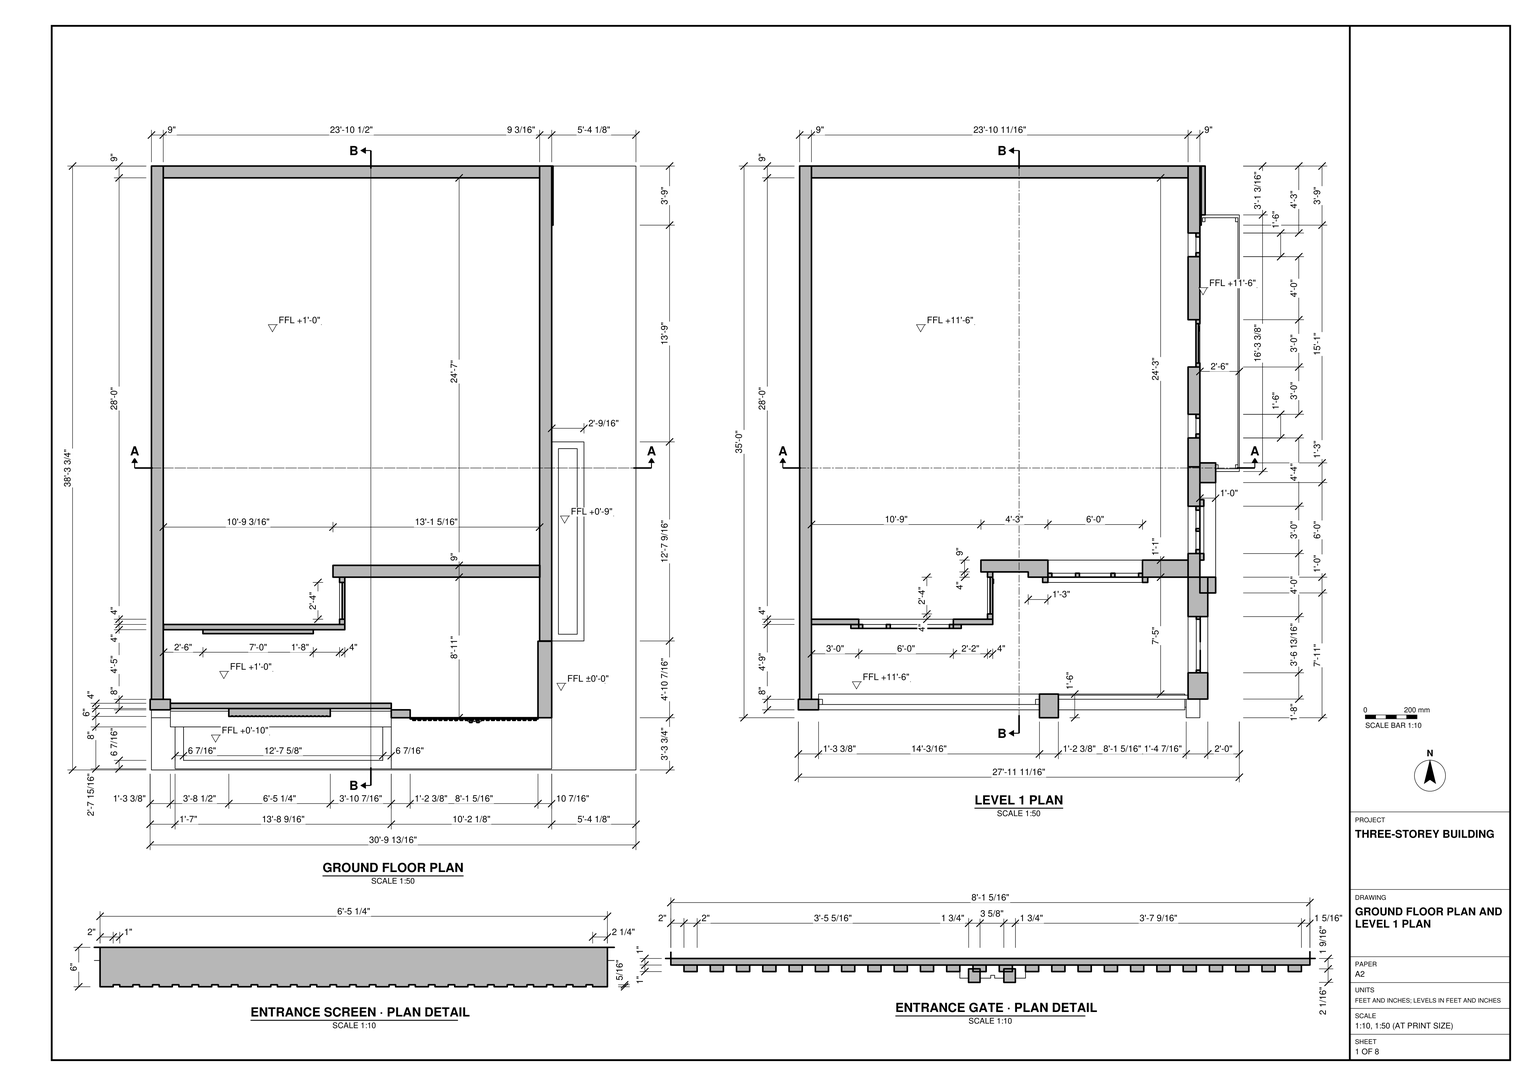
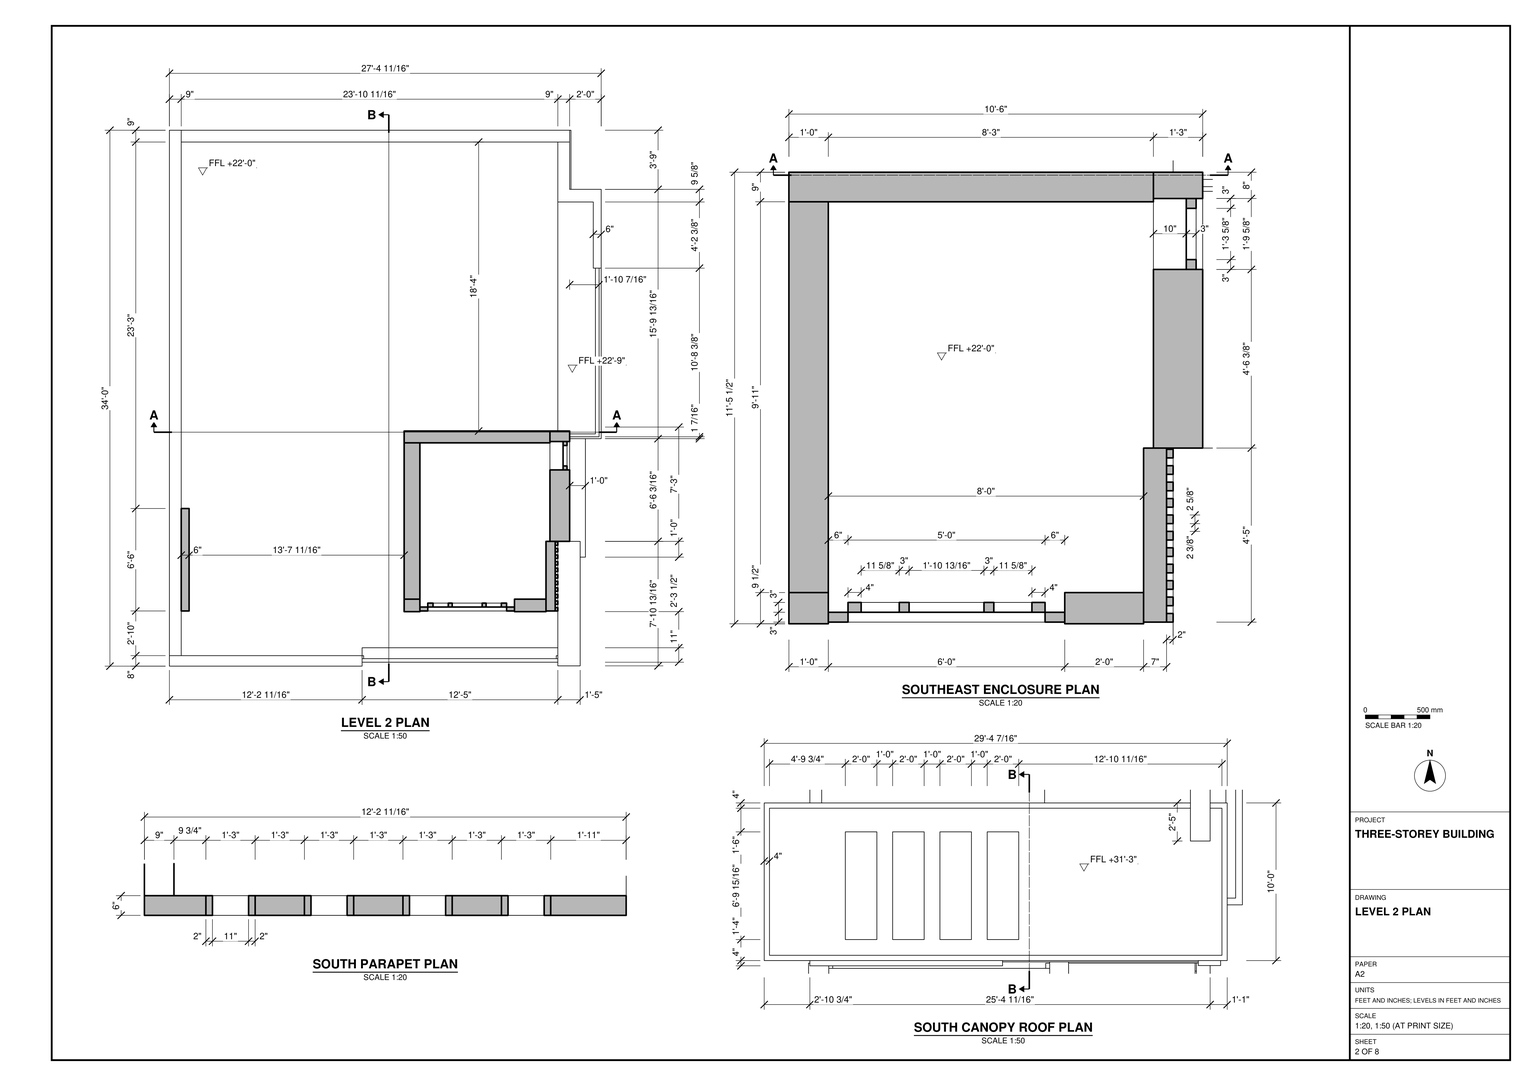
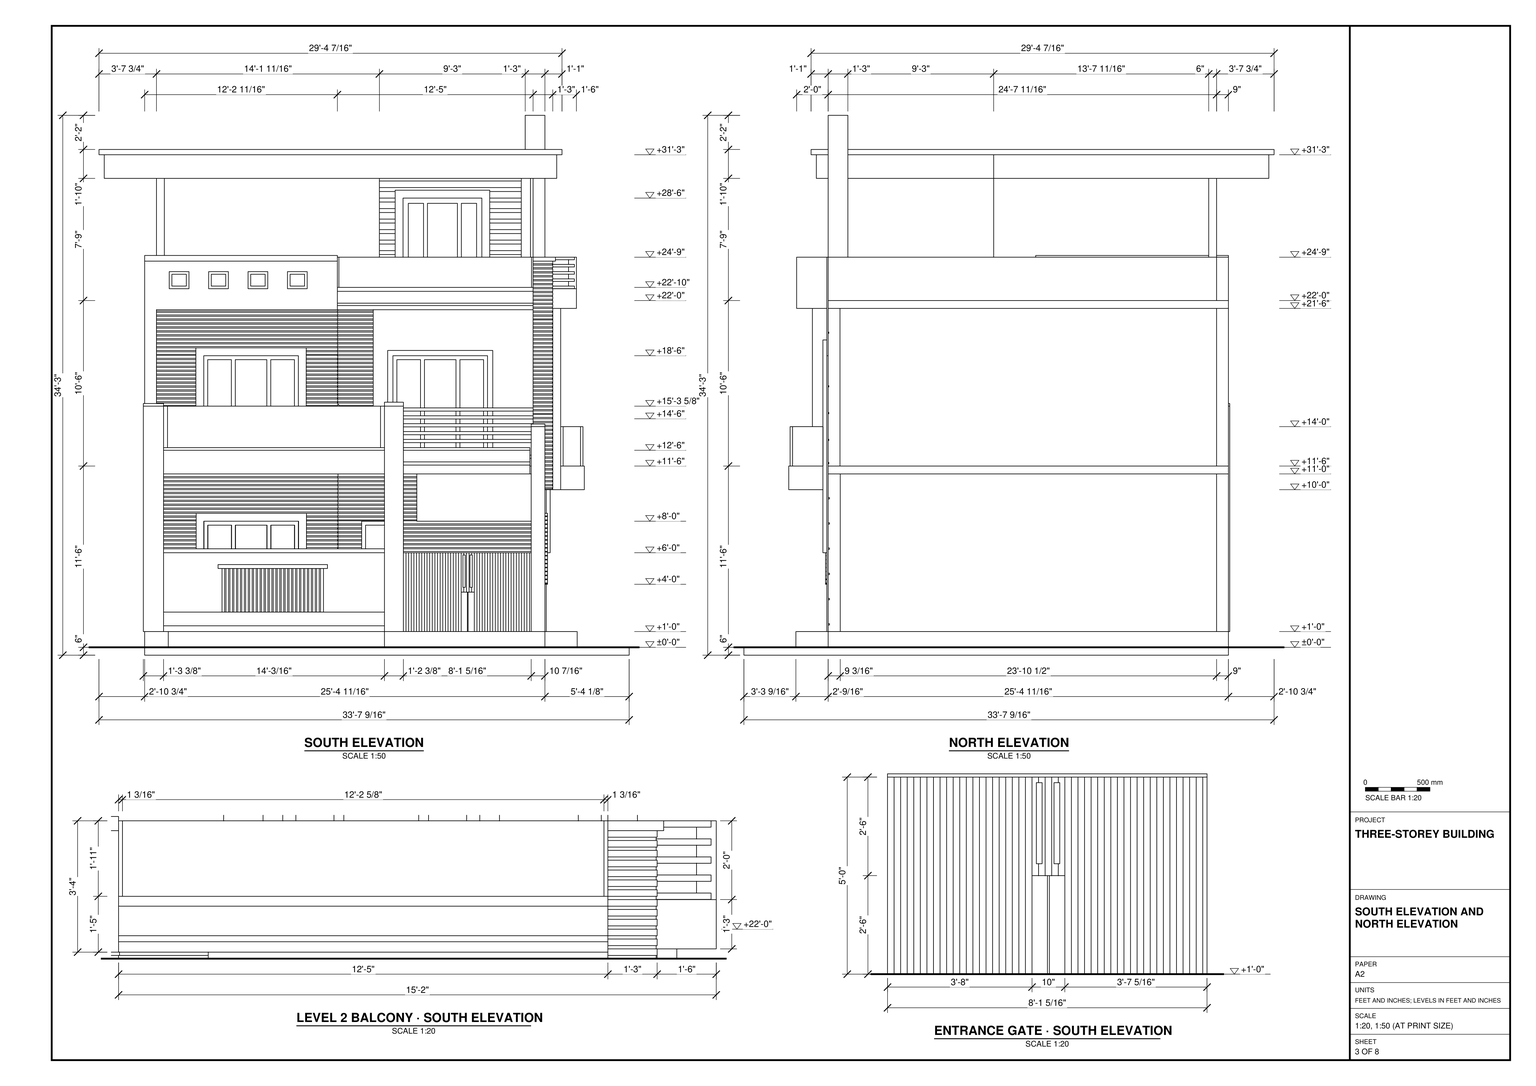
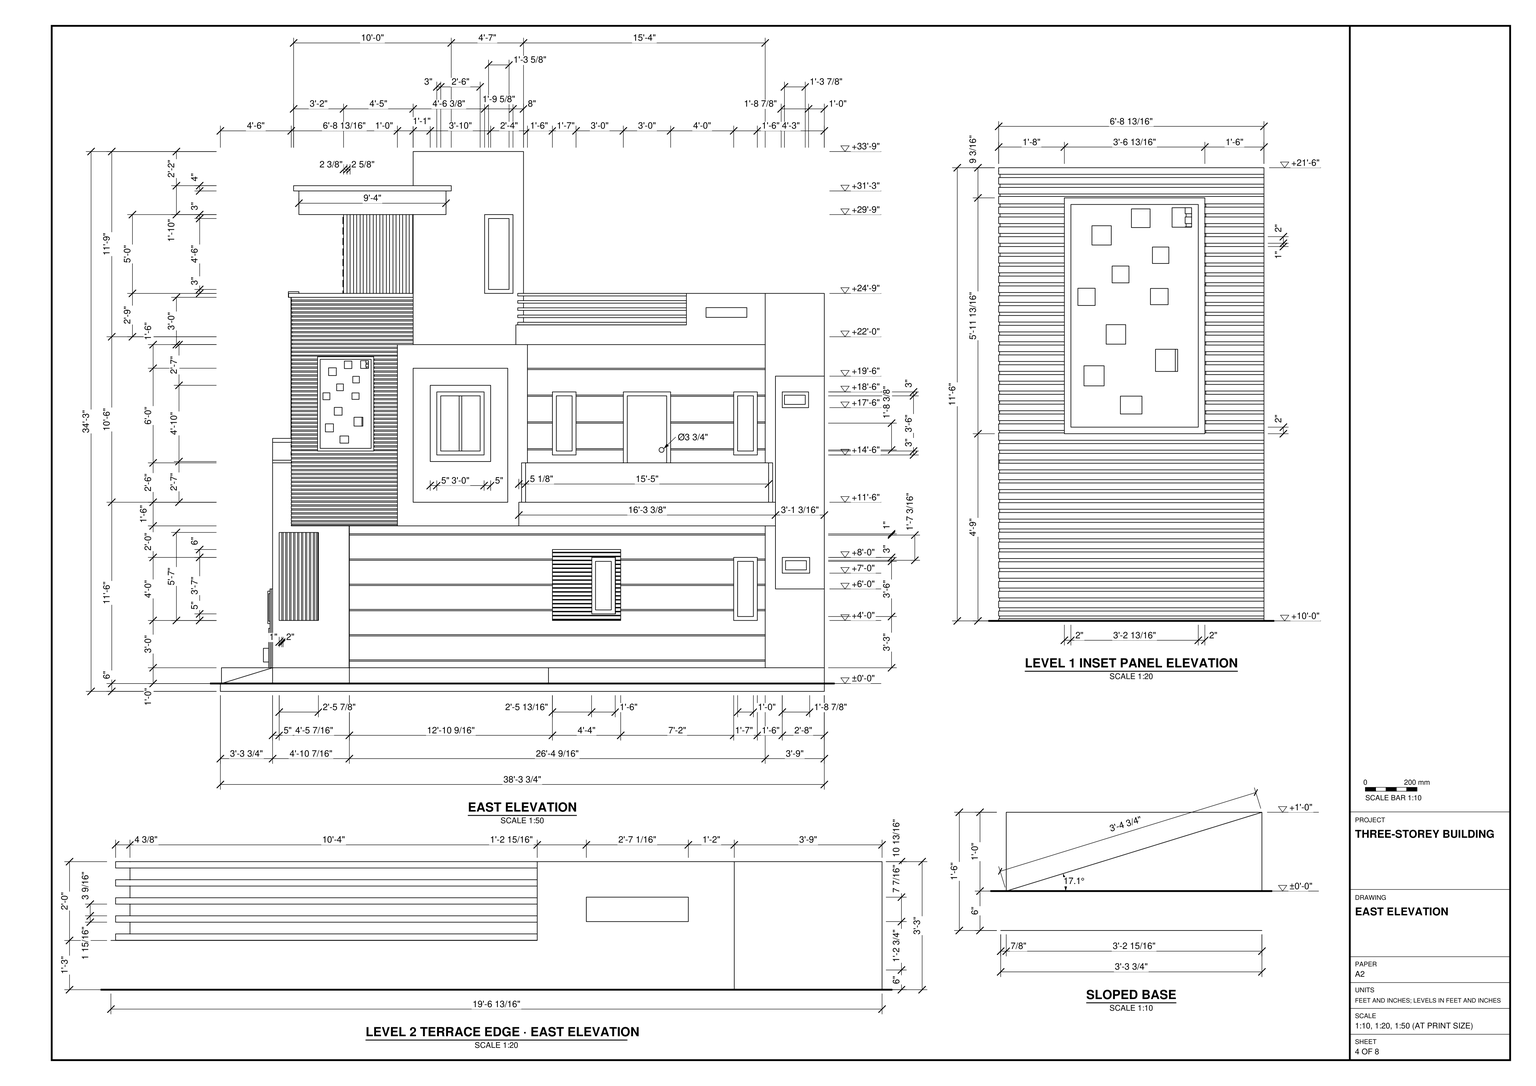
Build the three-storey building in SketchUp using the plans, elevations and details in task_files/diagram_01.pdf. Work in feet and inches. The overall model extents, including the base and projections, are 33'-7 9/16" wide, 38'-3 3/4" deep and 34'-3" high. Use the ground datum of ±0'-0", Level 1 at +11'-6" and Level 2 at +22'-0". Distinguish the raised ground floor at +1'-0" from the surrounding base.

Set out the floor slabs and walls from the plans, following the wall thicknesses and the stepped line of the south-facing rooms. Model the door and window openings with their frames and divisions. At the south entrance, distinguish the fixed screen from the two-leaf gate. Above them, form the balcony with its solid parapet and horizontal railing, and include the narrow balcony projecting on the east side. At Level 2, leave the terrace open around the southeast enclosure. Follow the details for the square openings in the south parapet and the long rectangular openings in the projecting canopy. Include stairs, built-in joinery and main furniture where shown on the sheets.

Keep walls, slabs, roof elements and each furniture or joinery piece in separate groups or components, and use components for repeated parts. Decor and loose items may be any suitable library components. Save one SketchUp model as output_files/three_storey_building_with_balconies_and_a_roof_terrace.skp.

# SketchUp Ruby script. Lengths in inches.
U = 1.inch
M = Sketchup.active_model
def pt(a) = Geom::Point3d.new(a.map { |v| v * U })
def face(e, loops, mat)
  f = e.add_face(loops[0].map { |a| pt(a) })
  loops[1..].each { |l| e.add_face(l.map { |a| pt(a) }).erase! }
  f.material = f.back_material = mat if mat
  f
end
# faces: each face lists its corners as indices into pts; further lists are holes
def faces(e, pts, list, mat = nil) = list.each { |f| face(e, (f[0].is_a?(Array) ? f : [f]).map { |l| l.map { |i| pts[i] } }, mat) }
# xy, xz, yz: faces in a plane at the given z, y or x. An outline is a flat list of corners, or four numbers for a rectangle; further outlines are holes
def ring(l) = l.size == 4 ? [[l[0], l[1]], [l[2], l[1]], [l[2], l[3]], [l[0], l[3]]] : l.each_slice(2).to_a
def flat(e, list, mat, &to3) = list.each { |f| face(e, (f[0].is_a?(Array) ? f : [f]).map { |l| ring(l).map { |u, v| to3.(u, v) } }, mat) }
def xy(e, z, list, mat = nil) = flat(e, list, mat) { |x, y| [x, y, z] }
def xz(e, y, list, mat = nil) = flat(e, list, mat) { |x, z| [x, y, z] }
def yz(e, x, list, mat = nil) = flat(e, list, mat) { |y, z| [x, y, z] }
def lines(e, pts, list) = list.each { |a, b| e.add_line(pt(pts[a]), pt(pts[b])) }
# prism: a flat outline (further loops are holes) pulled along v
def prism(e, loops, v, mat = nil)
  f = face(e, loops, mat); d = Geom::Vector3d.new(v.map { |x| x * U })
  f.pushpull(f.normal.samedirection?(d) ? d.length : -d.length)
end
def box(e, o, s, mat = nil) = prism(e, [[o, [o[0] + s[0], o[1], o[2]], [o[0] + s[0], o[1] + s[1], o[2]], [o[0], o[1] + s[1], o[2]]]], [0, 0, s[2]], mat)
def at(x, y, z, deg = 0) = Geom::Transformation.translation(pt([x, y, z])) * Geom::Transformation.rotation(ORIGIN, Z_AXIS, deg.degrees)
def axes(o, x, y, z) = Geom::Transformation.new([*x, 0, *y, 0, *z, 0, *pt(o).to_a, 1])
def part(name) = M.definitions.add(name)
# library, detail: a bought-in or finely detailed component or shape, given as its bounding box
def library(name, o, s) = part(name).tap { |d| box(d.entities, o, s) }
def detail(e, o, s) = box(e.add_group.entities, o, s)
def put(e, d, t, mat = nil) = e.add_instance(d, t).tap { |i| i.material = mat if mat }
def group(e, t, mat = nil) = e.add_group.tap { |g| g.transformation = t; g.material = mat if mat }.entities
root = M.entities
M.materials.add("[0133_Gray]").color = [128, 128, 128]
M.materials.add("[Aluminum]").color = [179, 179, 179]
M.materials.add("[Color I01]").color = [204, 204, 255]
M.materials.add("[Color M00]").color = [255, 255, 255]
M.materials.add("[Color M01]").color = [226, 226, 226]
M.materials.add("[Color M02]").color = [198, 198, 198]
M.materials.add("[Color M06]").color = [86, 86, 86]
M.materials.add("[Color M09]").color = [0, 0, 0]
M.materials.add("[Grass Dark Green]").color = [106, 157, 55]
M.materials.add("[Polished Concrete New]").color = [200, 200, 203]
M.materials.add("[Translucent Glass Gold]").color = [255, 150, 250]
M.materials["[Translucent Glass Gold]"].alpha = 0.6
M.materials.add("[Translucent Glass Gray]").color = [255, 255, 255]
M.materials["[Translucent Glass Gray]"].alpha = 0.5
M.materials.add("[Wood Bamboo]").color = [177, 105, 43]
M.materials.add("[Wood Cherry Original]").color = [152, 86, 42]
M.materials.add("[Wood Floor Dark]").color = [104, 64, 28]
M.materials.add("[Wood Floor Parquet]").color = [145, 89, 39]
M.materials.add("[Wood Veneer 01]").color = [120, 70, 37]
c1 = part("Group\#8")
prism(c1.entities,[[[2,20.86,12],[2,0,12],[2,0,0],[2,20.86,0]],[[2,18.36,2.5],[2,2.5,2.5],[2,2.5,9.5],[2,18.36,9.5]]],[-2,0,0])
c2 = part("Group\#11")
yz(c2.entities,0,[[0,0,15.86,7]])
c3 = part("Group\#21")
prism(c3.entities,[[[4,36,84],[4,0,84],[4,0,0],[4,36,0]],[[4,32,80],[4,32,4],[4,4,4],[4,4,80]]],[-4,0,0])
c4 = part("Group\#22")
box(c4.entities,[0,0,0],[2,28,76])
c5 = part("Group\#19")
prism(c5.entities,[[[0,0,120],[0,0,84],[9,0,84],[9,0,84.43],[8.7,0,84.43],[8.7,0,85.5],[9,0,85.5],[9,0,87],[8.7,0,87],[8.7,0,88],[9,0,88],[9,0,90],[8.7,0,90],[8.7,0,91],[9,0,91],[9,0,93],[8.7,0,93],[8.7,0,94],[9,0,94],[9,0,96],[8.7,0,96],[8.7,0,97],[9,0,97],[9,0,99],[8.7,0,99],[8.7,0,100],[9,0,100],[9,0,102],[8.7,0,102],[8.7,0,103],[9,0,103],[9,0,105],[8.7,0,105],[8.7,0,106],[9,0,106],[9,0,108],[8.7,0,108],[8.7,0,109],[9,0,109],[9,0,111],[8.7,0,111],[8.7,0,112],[9,0,112],[9,0,114],[8.7,0,114],[8.7,0,115],[9,0,115],[9,0,117],[8.7,0,117],[8.7,0,118],[9,0,118],[9,0,120]]],[0,36,0])
c6 = library("Group\#18",[54,0,0],[138,4,120])
c7 = part("Group\#23")
prism(c7.entities,[[[0,3,0],[0,3,60],[84,3,60],[84,3,0]],[[6,3,54],[6,3,6],[78,3,6],[78,3,54]]],[0,-3,0])
c8 = part("Group\#24")
prism(c8.entities,[[[72,3,0],[0,3,0],[0,3,48],[72,3,48]],[[24,3,3],[48,3,3],[48,3,45],[24,3,45]],[[21,3,3],[21,3,45],[3,3,45],[3,3,3]],[[51,3,45],[51,3,3],[69,3,3],[69,3,45]]],[0,-3,0])
c9 = part("Group\#25")
xz(c9.entities,0,[[0,0,18,42]])
c10 = part("Group\#26")
xz(c10.entities,0,[[0,0,24,42]])
c11 = part("Group\#27")
xz(c11.entities,0,[[0,0,18,42]])
c12 = library("Group\#17",[-4.9,0,0],[157.5,9,120])
c13 = library("Group\#33",[0,0,-8],[77.25,6,33.2])
c14 = library("Group\#46",[0,0.17,0],[5,52,54])
c15 = part("Group\#60")
box(c15.entities,[0,0,0],[1.875,3.0625,30])
c16 = library("Group\#64",[0,1.46,-18],[15,92.79,174])
c17 = library("Group\#39",[0,-4,0],[157.69,13,120])
c18 = part("Group\#70")
box(c18.entities,[0,0,0],[3,3.9375,31.6])
c19 = part("Group\#72")
box(c19.entities,[0,0,0],[98.74,3.125,2.4375])
c20 = part("Group\#80")
box(c20.entities,[0,0,0],[1.1875,2.25,23])
c21 = part("Group\#86")
prism(c21.entities,[[[19.61,128.38,0],[22.42,128.38,0],[22.42,0,0],[0,0,0],[0,2.2,0],[19.61,2.2,0]]],[0,0,1.9375])
c22 = part("Group\#90")
box(c22.entities,[0,0,0],[2,2.63,93])
c23 = library("Group\#91",[0,-0.5,0],[108,9.5,93])
c24 = part("Group\#101")
box(c24.entities,[0,0,0],[2,1,60])
c25 = part("Group\#108")
prism(c25.entities,[[[1.75,2.0625,22.86],[1.75,2.0625,24.6875],[1.75,0,24.6875],[1.75,0,0],[1.75,2.0625,0],[1.75,2.0625,1.76],[1.75,0.76,1.76],[1.75,0.76,22.86]]],[-1.75,0,0])
box(root,[43.75,450.78,18],[286.5,9,120])
box(root,[43.75,450.78,144],[286.69,9,120])
box(root,[33.75,45.78,189.6],[15.4,8,2])
box(root,[329.01,39.78,174],[10.43,14.2,2])
xy(root,6,[[339.44,98.2,364.01,249.78]])
xy(root,15,[[344.58,103.33,358.875,244.64]],"[Grass Dark Green]")
xy(root,18,[[[339.44,98.2,364.01,249.78],[344.58,103.33,358.875,244.64]]],"[Polished Concrete New]")
xz(root,98.2,[[339.44,6,364.01,18]],"[Polished Concrete New]")
xz(root,103.33,[[344.58,15,358.875,18]])
xz(root,244.64,[[344.58,15,358.875,18]])
xz(root,249.78,[[339.44,6,364.01,18]])
yz(root,339.44,[[98.2,6,249.78,18]])
yz(root,339.69,[[[75.99,185,114.78,252.8125],[101.75,201.96,108.5,208.71],[79.97,197.57,86.1,203.69],[91.0625,189.01,97.625,194.45],[106.8,245.89,112.74,251.83],[86.73,210.27,92.67,216.21],[82.4,240.46,88.27,246.33],[94.42,245.78,100.11,251.46],[78.11,222.05,83.36,227.3],[100.21,222.3,105.59,227.24],[88.54,228.9375,93.66,234.0625],[100.8125,234.85,105.8125,239.85]]],"[Wood Floor Parquet]")
yz(root,344.58,[[103.33,15,244.64,18]])
yz(root,358.875,[[103.33,15,244.64,18]])
yz(root,364.01,[[98.2,6,249.78,18]],"[Polished Concrete New]")
p = [[339.44,55.36,138],[339.44,55.36,126],[345.44,134.78,264],[345.44,134.78,126]]
lines(root,p,[[0,1],[2,3]])
g1 = group(root,at(-197.67,12,0))
box(g1,[232.42,-12,0],[368.83,459.78,6])
g2 = group(root,at(336.44,390.78,54),"[Color M09]")
prism(g2,[[[0,0,48],[0,18,48],[0,18,0],[0,0,0]],[[0,3,3],[0,15,3],[0,15,45],[0,3,45]]],[3,0,0])
put(root,c1,at(337.44,427.78,90),"[Color M09]")
g3 = group(root,at(339.44,393.78,57),"[Translucent Glass Gray]")
yz(g3,0,[[0,0,12,42]])
put(root,c2,at(339.44,430.28,92.5),"[Translucent Glass Gold]")
g4 = group(root,at(339.44,414.78,18),"[Color M02]")
xy(g4,0,[[0,0,1,45]])
xy(g4,72,[[0,13,1,33.86]])
xy(g4,84,[[0,13,1,33.86]])
xy(g4,198,[[0,13,1,33]])
xy(g4,210,[[0,13,1,33]])
xy(g4,285,[[0,0,1,45]])
xz(g4,0,[[0,0,1,285]])
xz(g4,13,[[0,72,1,84],[0,198,1,210]])
xz(g4,33,[[0,198,1,210]])
xz(g4,33.86,[[0,72,1,84]])
xz(g4,45,[[0,0,1,210],[0,210,1,285]])
yz(g4,0,[[[0,0,0,285,45,285,45,210,13,210,13,198,33,198,33,210,45,210,45,0],[13,72,33.86,84]]])
yz(g4,1,[[[0,0,45,285],[13,72,33.86,84],[13,198,33,210]]])
g5 = group(root,at(340.44,422.58,78),"[Color M02]")
xy(g5,0,[[0,0,3,37.2]])
xy(g5,12,[[0,5.2,3,26.06]])
xy(g5,24,[[0,5.2,3,26.06]])
xy(g5,138,[[0,5.2,3,25.2]])
xy(g5,150,[[0,5.2,3,25.2]])
xy(g5,162,[[0,0,3,37.2]])
xz(g5,0,[[0,0,3,150],[0,150,3,162]])
xz(g5,5.2,[[0,12,3,24],[0,138,3,150]])
xz(g5,25.2,[[0,138,3,150]])
xz(g5,26.06,[[0,12,3,24]])
xz(g5,37.2,[[0,0,3,162]])
yz(g5,0,[[[0,0,0,150,5.2,150,5.2,138,25.2,138,25.2,150,0,150,0,162,37.2,162,37.2,0],[5.2,12,26.06,24]]])
yz(g5,3,[[[0,0,37.2,162],[5.2,12,26.06,24],[5.2,138,25.2,150]]])
g6 = group(root,at(331.35,49.4,18),"[Color M06]")
prism(g6,[[[-2.35,48.61,0],[-2.35,48.61,120],[-2.35,5.96,120],[-2.35,5.96,156],[-2.35,-9.625,156],[-2.35,-9.625,0]],[[-2.35,25.24,103],[-2.35,25.24,36],[-2.35,-4.625,36],[-2.35,-4.625,103]]],[10.4375,0,0])
put(root,c3,at(177.94,110.78,18),"[Wood Veneer 01]")
put(root,c4,at(179.94,114.78,22),"[Wood Bamboo]")
g7 = group(root,at(217.31,47.78,18),"[Color M06]")
prism(g7,[[[0,-2,0],[0,-8,0],[0,-8,171.6],[0,10,171.6],[0,10,120.5],[0,-2,120.5]]],[14.4,0,0])
g8 = group(root,at(-140.56,99.78,6),"[Polished Concrete New]")
box(g8,[175.31,-60,0],[304.69,420,12])
put(root,c5,at(172.94,110.78,18),"[Color I01]")
put(root,c6,at(-10.06,106.78,18),"[Color I01]")
put(root,c7,at(73.94,103.78,48))
put(root,c8,at(79.75,103.78,54),"[Color M09]")
put(root,c9,at(130.94,103.78,57),"[Translucent Glass Gold]")
put(root,c10,at(103.94,103.78,57),"[Translucent Glass Gold]")
put(root,c11,at(82.94,103.78,57),"[Translucent Glass Gold]")
g9 = group(root,at(34.75,128.78,18),"[Color M06]")
box(g9,[0,-75,0],[9,406,120])
g10 = group(root,at(34.75,47.78,18),"[Color M06]")
box(g10,[-1,-2,0],[15.4,8,171.6])
g11 = group(root,at(34.75,105.78,138))
prism(g11,[[[0,-58,0],[0,354,0],[304.69,354,0],[304.69,-50.42,0],[295.69,-50.42,0],[295.69,-58,0]]],[0,0,6])
put(root,c12,at(177.85,146.78,18),"[Color I01]")
g12 = group(root,at(49.15,44.78,18),"[Wood Floor Dark]")
box(g12,[0,2,0],[168.16,4,60])
g13 = group(root,at(49.15,44.78,78))
box(g13,[0,0,0],[168.16,6,3])
g14 = group(root,at(49.15,32.78,18),"[Color M02]")
box(g14,[0,0,4.375],[168.16,12,10.42])
put(root,c13,at(93.64,40.78,40.8),"[Color I01]")
g15 = group(root,at(90.64,40.78,66))
box(g15,[0,0,0],[83.25,6,3])
g16 = group(root,at(24.75,45.78,138),"[Color M06]")
xy(g16,0,[[24.4,0,303.25,2]])
xy(g16,6,[[24.4,2,303.25,12]])
xy(g16,6.72,[[206.96,0,303.25,2]],"[Color M00]")
xy(g16,9.15,[[206.96,0,303.25,2]],"[Color M00]")
xy(g16,18,[[24.4,0,303.25,12]])
xz(g16,0,[[24.4,0,303.25,0,303.25,6.72,206.96,6.72,206.96,9.15,303.25,9.15,303.25,18,24.4,18]])
xz(g16,2,[[24.4,0,303.25,6]])
xz(g16,2,[[206.96,6.72,303.25,9.15]],"[Color M00]")
xz(g16,12,[[24.4,6,303.25,18]])
yz(g16,24.4,[[0,0,0,18,12,18,12,6,2,6,2,0]])
yz(g16,206.96,[[0,6.72,2,9.15]])
yz(g16,303.25,[[0,0,2,0,2,6,12,6,12,18,0,18,0,9.15,2,9.15,2,6.72,0,6.72]])
g17 = group(root,at(199.94,146.78,54),"[Color M09]")
prism(g17,[[[24,0,48],[0,0,48],[0,0,0],[24,0,0]],[[3,0,3],[3,0,45],[21,0,45],[21,0,3]]],[0,3,0])
g18 = group(root,at(202.94,146.78,57),"[Translucent Glass Gold]")
xz(g18,0,[[0,0,18,42]])
g19 = group(root,at(241.94,122.78,102))
xy(g19,0,[[0,-24.77,88.5,24]])
xy(g19,36,[[0,-24.77,88.5,24]])
xz(g19,-24.77,[[0,0,88.5,36]],"[Wood Floor Dark]")
xz(g19,24,[[0,0,88.5,36]])
yz(g19,0,[[-24.77,0,24,36]])
yz(g19,88.5,[[-24.77,0,24,36]])
g20 = group(root,at(223.75,146.78,150),"[Color M09]")
prism(g20,[[[0,3,78],[72,3,78],[72,3,0],[0,3,0]],[[48,3,75],[24,3,75],[24,3,3],[48,3,3]],[[21,3,3],[21,3,75],[3,3,75],[3,3,3]],[[69,3,75],[51,3,75],[51,3,3],[69,3,3]]],[0,-3,0])
g21 = group(root,at(226.75,146.78,153),"[Translucent Glass Gold]")
xz(g21,0,[[0,0,18,72]])
put(root,c1,at(337.44,426.92,216),"[Color M09]")
put(root,c2,at(339.44,429.42,218.5),"[Translucent Glass Gold]")
put(root,c14,at(336.44,252.61,54),"[Color I01]")
g22 = group(root,at(330.25,99.78,18),"[0133_Gray]")
xy(g22,0,[[0,-1.58,9.19,360]])
xy(g22,5,[[8.19,-1.58,9.19,360]])
xy(g22,6,[[8.19,-1.58,9.19,360]])
xy(g22,24.2,[[8.19,-1.58,9.19,360]])
xy(g22,25.2,[[8.19,-1.58,9.19,360]])
xy(g22,36,[[0,291,9.19,309]])
xy(g22,41,[[0,183,9.19,201]])
xy(g22,43.4,[[8.19,-1.58,9.19,183],[8.19,201,9.19,291],[8.19,309,9.19,360]])
xy(g22,44.4,[[8.19,-1.58,9.19,183],[8.19,201,9.19,291],[8.19,309,9.19,360]])
xy(g22,62.6,[[8.19,-1.58,9.19,183],[8.19,201,9.19,291],[8.19,309,9.19,360]])
xy(g22,63.6,[[8.19,-1.58,9.19,183],[8.19,201,9.19,291],[8.19,309,9.19,360]])
xy(g22,72,[[0,328,9.19,348.86]])
xy(g22,81.8,[[8.19,-1.58,9.19,183],[8.19,201,9.19,291],[8.19,309,9.19,328],[8.19,348.86,9.19,360]])
xy(g22,82.8,[[8.19,-1.58,9.19,183],[8.19,201,9.19,291],[8.19,309,9.19,328],[8.19,348.86,9.19,360]])
xy(g22,84,[[0,183,9.19,201],[0,291,9.19,309],[0,328,9.19,348.86]])
xy(g22,101,[[8.19,-1.58,9.19,360]])
xy(g22,102,[[8.19,-1.58,9.19,360]])
xy(g22,120,[[0,-1.58,9.19,360]])
xz(g22,-1.58,[[0,0,9.19,0,9.19,5,8.19,5,8.19,6,9.19,6,9.19,24.2,8.19,24.2,8.19,25.2,9.19,25.2,9.19,43.4,8.19,43.4,8.19,44.4,9.19,44.4,9.19,62.6,8.19,62.6,8.19,63.6,9.19,63.6,9.19,81.8,8.19,81.8,8.19,82.8,9.19,82.8,9.19,101,8.19,101,8.19,102,9.19,102,9.19,120,0,120]])
xz(g22,183,[[0,41,0,84,9.19,84,9.19,82.8,8.19,82.8,8.19,81.8,9.19,81.8,9.19,63.6,8.19,63.6,8.19,62.6,9.19,62.6,9.19,44.4,8.19,44.4,8.19,43.4,9.19,43.4,9.19,41]])
xz(g22,201,[[0,41,9.19,41,9.19,43.4,8.19,43.4,8.19,44.4,9.19,44.4,9.19,62.6,8.19,62.6,8.19,63.6,9.19,63.6,9.19,81.8,8.19,81.8,8.19,82.8,9.19,82.8,9.19,84,0,84]])
xz(g22,291,[[0,36,0,84,9.19,84,9.19,82.8,8.19,82.8,8.19,81.8,9.19,81.8,9.19,63.6,8.19,63.6,8.19,62.6,9.19,62.6,9.19,44.4,8.19,44.4,8.19,43.4,9.19,43.4,9.19,36]])
xz(g22,309,[[0,36,9.19,36,9.19,43.4,8.19,43.4,8.19,44.4,9.19,44.4,9.19,62.6,8.19,62.6,8.19,63.6,9.19,63.6,9.19,81.8,8.19,81.8,8.19,82.8,9.19,82.8,9.19,84,0,84]])
xz(g22,328,[[0,72,0,84,9.19,84,9.19,82.8,8.19,82.8,8.19,81.8,9.19,81.8,9.19,72]])
xz(g22,348.86,[[0,72,9.19,72,9.19,81.8,8.19,81.8,8.19,82.8,9.19,82.8,9.19,84,0,84]])
xz(g22,360,[[0,0,0,120,9.19,120,9.19,102,8.19,102,8.19,101,9.19,101,9.19,82.8,8.19,82.8,8.19,81.8,9.19,81.8,9.19,63.6,8.19,63.6,8.19,62.6,9.19,62.6,9.19,44.4,8.19,44.4,8.19,43.4,9.19,43.4,9.19,25.2,8.19,25.2,8.19,24.2,9.19,24.2,9.19,6,8.19,6,8.19,5,9.19,5,9.19,0]])
yz(g22,0,[[[-1.58,0,360,120],[291,36,309,84],[183,41,201,84],[328,72,348.86,84]]])
yz(g22,8.19,[[-1.58,5,360,6],[-1.58,24.2,360,25.2],[-1.58,43.4,183,44.4],[201,43.4,291,44.4],[309,43.4,360,44.4],
  [-1.58,62.6,183,63.6],[201,62.6,291,63.6],[309,62.6,360,63.6],[-1.58,81.8,183,82.8],[201,81.8,291,82.8],
  [309,81.8,328,82.8],[348.86,81.8,360,82.8],[-1.58,101,360,102]])
yz(g22,9.19,[[-1.58,0,360,5],[-1.58,6,360,24.2],[-1.58,25.2,360,25.2,360,43.4,309,43.4,309,36,291,36,291,43.4,201,43.4,201,41,183,41,183,43.4,-1.58,43.4],[-1.58,44.4,183,62.6],[201,44.4,291,62.6],
  [309,44.4,360,62.6],[-1.58,63.6,183,81.8],[201,63.6,291,81.8],[309,63.6,360,63.6,360,81.8,348.86,81.8,348.86,72,328,72,328,81.8,309,81.8],[-1.58,82.8,183,82.8,183,84,201,84,201,82.8,291,82.8,291,84,309,84,309,82.8,328,82.8,328,84,348.86,84,348.86,82.8,360,82.8,360,101,-1.58,101],
  [-1.58,102,360,120]])
g23 = group(root,at(330.44,188.78,144),"[0133_Gray]")
xy(g23,0,[[0,42,9,118],[0,154,9,271]])
xy(g23,1.68,[[8.5,42,9,118],[8.5,154,9,271]])
xy(g23,2.82,[[8.5,42,9,118],[8.5,154,9,271]])
xy(g23,19.4,[[8.5,42,9,118],[8.5,154,9,271]])
xy(g23,20.4,[[8.5,42,9,118],[8.5,154,9,271]])
xy(g23,36,[[0,64,9,82],[0,202,9,220]])
xy(g23,39.8,[[8.5,42,9,64],[8.5,82,9,118],[8.5,154,9,202],[8.5,220,9,271]])
xy(g23,40.8,[[8.5,42,9,64],[8.5,82,9,118],[8.5,154,9,202],[8.5,220,9,271]])
xy(g23,60.2,[[8.5,42,9,64],[8.5,82,9,118],[8.5,154,9,202],[8.5,220,9,271]])
xy(g23,61.2,[[8.5,42,9,64],[8.5,82,9,118],[8.5,154,9,202],[8.5,220,9,271]])
xy(g23,72,[[0,239,9,259]])
xy(g23,80.6,[[8.5,42,9,64],[8.5,82,9,118],[8.5,154,9,202],[8.5,220,9,239]])
xy(g23,81.6,[[8.5,42,9,64],[8.5,82,9,118],[8.5,154,9,202],[8.5,220,9,239]])
xy(g23,84,[[0,64,9,82],[0,118,9,154],[0,202,9,220],[0,239,9,259]])
xy(g23,101,[[8.5,42,9,271]])
xy(g23,102,[[8.5,42,9,271]])
xy(g23,120,[[0,42,9,271]])
xz(g23,42,[[0,0,9,0,9,1.68,8.5,1.68,8.5,2.82,9,2.82,9,19.4,8.5,19.4,8.5,20.4,9,20.4,9,39.8,8.5,39.8,8.5,40.8,9,40.8,9,60.2,8.5,60.2,8.5,61.2,9,61.2,9,80.6,8.5,80.6,8.5,81.6,9,81.6,9,101,8.5,101,8.5,102,9,102,9,120,0,120]])
xz(g23,64,[[0,36,0,84,9,84,9,81.6,8.5,81.6,8.5,80.6,9,80.6,9,61.2,8.5,61.2,8.5,60.2,9,60.2,9,40.8,8.5,40.8,8.5,39.8,9,39.8,9,36]])
xz(g23,82,[[0,36,9,36,9,39.8,8.5,39.8,8.5,40.8,9,40.8,9,60.2,8.5,60.2,8.5,61.2,9,61.2,9,80.6,8.5,80.6,8.5,81.6,9,81.6,9,84,0,84]])
xz(g23,118,[[0,0,0,84,9,84,9,81.6,8.5,81.6,8.5,80.6,9,80.6,9,61.2,8.5,61.2,8.5,60.2,9,60.2,9,40.8,8.5,40.8,8.5,39.8,9,39.8,9,20.4,8.5,20.4,8.5,19.4,9,19.4,9,2.82,8.5,2.82,8.5,1.68,9,1.68,9,0]])
xz(g23,154,[[0,0,9,0,9,1.68,8.5,1.68,8.5,2.82,9,2.82,9,19.4,8.5,19.4,8.5,20.4,9,20.4,9,39.8,8.5,39.8,8.5,40.8,9,40.8,9,60.2,8.5,60.2,8.5,61.2,9,61.2,9,80.6,8.5,80.6,8.5,81.6,9,81.6,9,84,0,84]])
xz(g23,202,[[0,36,0,84,9,84,9,81.6,8.5,81.6,8.5,80.6,9,80.6,9,61.2,8.5,61.2,8.5,60.2,9,60.2,9,40.8,8.5,40.8,8.5,39.8,9,39.8,9,36]])
xz(g23,220,[[0,36,9,36,9,39.8,8.5,39.8,8.5,40.8,9,40.8,9,60.2,8.5,60.2,8.5,61.2,9,61.2,9,80.6,8.5,80.6,8.5,81.6,9,81.6,9,84,0,84]])
xz(g23,239,[[0,72,0,84,9,84,9,81.6,8.5,81.6,8.5,80.6,9,80.6,9,72]])
xz(g23,259,[[0,72,9,84]])
xz(g23,271,[[0,0,0,120,9,120,9,102,8.5,102,8.5,101,9,101,9,61.2,8.5,61.2,8.5,60.2,9,60.2,9,40.8,8.5,40.8,8.5,39.8,9,39.8,9,20.4,8.5,20.4,8.5,19.4,9,19.4,9,2.82,8.5,2.82,8.5,1.68,9,1.68,9,0]])
yz(g23,0,[[[42,0,42,120,271,120,271,0,154,0,154,84,118,84,118,0],[202,36,220,84],[64,36,82,84],[239,72,259,84]]])
yz(g23,8.5,[[42,1.68,118,2.82],[154,1.68,271,2.82],[42,19.4,118,20.4],[154,19.4,271,20.4],[42,39.8,64,40.8],
  [82,39.8,118,40.8],[154,39.8,202,40.8],[220,39.8,271,40.8],[42,60.2,64,61.2],[82,60.2,118,61.2],
  [154,60.2,202,61.2],[220,60.2,271,61.2],[42,80.6,64,81.6],[82,80.6,118,81.6],[154,80.6,202,81.6],
  [220,80.6,239,81.6],[42,101,271,102]])
yz(g23,9,[[42,0,118,1.68],[154,0,271,1.68],[42,2.82,118,19.4],[154,2.82,271,19.4],[42,20.4,118,20.4,118,39.8,82,39.8,82,36,64,36,64,39.8,42,39.8],
  [154,20.4,271,20.4,271,39.8,220,39.8,220,36,202,36,202,39.8,154,39.8],[42,40.8,64,60.2],[82,40.8,118,60.2],[154,40.8,202,60.2],[220,40.8,271,60.2],
  [220,61.2,271,61.2,271,101,42,101,42,81.6,64,81.6,64,84,82,84,82,81.6,118,81.6,118,84,154,84,154,81.6,202,81.6,202,84,220,84,220,81.6,239,81.6,239,84,259,84,259,72,239,72,239,80.6,220,80.6],[42,61.2,64,80.6],[82,61.2,118,80.6],[154,61.2,202,80.6],[42,102,271,120]])
g24 = group(root,at(336.44,390.78,180),"[Color M09]")
prism(g24,[[[0,0,48],[0,18,48],[0,18,0],[0,0,0]],[[0,15,3],[0,15,45],[0,3,45],[0,3,3]]],[3,0,0])
g25 = group(root,at(339.44,393.78,183),"[Translucent Glass Gray]")
yz(g25,0,[[0,0,12,42]])
g26 = group(root,at(336.44,306.78,144),"[Wood Veneer 01]")
prism(g26,[[[3,0,0],[3,36,0],[3,36,84],[3,0,84]],[[3,3,3],[3,3,81],[3,33,81],[3,33,3]]],[-3,0,0])
g27 = group(root,at(336.44,309.78,147),"[Wood Bamboo]")
box(g27,[0,0,0],[2,30,78])
g28 = group(root,at(336.44,252.78,180),"[Color M09]")
prism(g28,[[[0,0,48],[0,18,48],[0,18,0],[0,0,0]],[[0,3,45],[0,3,3],[0,15,3],[0,15,45]]],[3,0,0])
g29 = group(root,at(339.44,255.78,183),"[Translucent Glass Gray]")
yz(g29,0,[[0,0,12,42]])
g30 = group(root,at(330.44,158.78,144),"[Wood Floor Dark]")
xy(g30,0,[[0,-12,9,72]])
xy(g30,36,[[0,6,9,42]])
xy(g30,84,[[0,6,9,42]])
xy(g30,126,[[-6,-12,0,72]])
xy(g30,159,[[-6,42.4,9,64]],"[Wood Floor Dark]")
xy(g30,219,[[-6,42.4,9,64]],"[Wood Floor Dark]")
xy(g30,267,[[-6,-12,9,72]])
xz(g30,-12,[[0,0,9,0,9,267,-6,267,-6,126,0,126]])
xz(g30,6,[[0,36,9,84]])
xz(g30,42,[[0,36,9,84]])
xz(g30,42.4,[[-6,159,9,219]],"[Wood Floor Dark]")
xz(g30,64,[[-6,159,9,219]],"[Wood Floor Dark]")
xz(g30,72,[[0,0,0,126,-6,126,-6,267,9,267,9,0]])
yz(g30,-6,[[[-12,126,72,267],[42.4,159,64,219]]])
yz(g30,0,[[[-12,0,72,126],[6,36,42,84]]])
yz(g30,9,[[[-12,0,72,267],[6,36,42,84],[42.4,159,64,219]]],"[Wood Floor Dark]")
g31 = group(root,at(339.44,159.78,175))
prism(g31,[[[3,0,58],[3,0,0],[3,46,0],[3,46,58]],[[3,5,53],[3,41,53],[3,41,5],[3,5,5]]],[-3,0,0])
g32 = group(root,at(336.44,164.78,180),"[Color M09]")
prism(g32,[[[0,0,48],[0,36,48],[0,36,0],[0,0,0]],[[0,19,45],[0,19,3],[0,33,3],[0,33,45]],[[0,17,45],[0,3,45],[0,3,3],[0,17,3]]],[3,0,0])
g33 = group(root,at(339.44,167.78,183),"[Translucent Glass Gray]")
yz(g33,0,[[0,0,30,42]])
g34 = group(root,at(339.44,134.78,144))
prism(g34,[[[0,99,120],[0,99,-18],[0,0,-18],[0,0,120]],[[0,12,102],[0,12,0],[0,84,0],[0,84,102]]],[12,0,0])
g35 = group(root,at(339.44,227.21,126),"[Color M06]")
box(g35,[0,0,0],[30,195.36,18])
put(root,c15,at(366.53,229.3,144),"[Color M09]")
put(root,c15,at(366.53,417.37,144),"[Color M09]")
put(root,c15,at(341.47,417.37,144),"[Color M09]")
g36 = group(root,at(368.41,232.37,144),"[Translucent Glass Gray]")
yz(g36,0,[[0,0,185,30]])
g37 = group(root,at(343.35,420.43,144),"[Translucent Glass Gray]")
xz(g37,0,[[0,0,23.1875,30]])
put(root,c15,at(351.44,229.3,144),"[Color M09]")
g38 = group(root,at(353.32,229.3,144),"[Translucent Glass Gray]")
xz(g38,0,[[0,0,13.21,30]])
put(root,c16,at(330.44,52.53,144),"[Color I01]")
g39 = group(root,at(336.69,73.99,183),"[Wood Cherry Original]")
prism(g39,[[[0,0,71.8125],[0,42.79,71.8125],[0,42.79,0],[0,0,0]],[[0,2,69.8125],[0,2,2],[0,40.79,2],[0,40.79,69.8125]]],[3,0,0])
g40 = group(root,at(43.75,107.78,144))
g41 = group(g40,at(176,35,2))
prism(g41,[[[80,0,0],[80,0,86],[0,0,86],[0,0,0]],[[4,0,4],[4,0,82],[76,0,82],[76,0,4]]],[0,4,0])
put(g40,c8,at(36,0,36),"[Color M09]")
put(g40,c6,at(-54,3,0),"[Color I01]")
put(g40,c5,at(129,7,0),"[Color I01]")
put(g40,c17,at(129,43,0),"[Color I01]")
put(g40,c3,at(134,7,0),"[Wood Veneer 01]")
put(g40,c10,at(60,0,39),"[Translucent Glass Gold]")
put(g40,c9,at(87,0,39),"[Translucent Glass Gold]")
put(g40,c11,at(39,0,39),"[Translucent Glass Gold]")
g42 = group(g40,at(231,39,9),"[Translucent Glass Gold]")
xz(g42,0,[[0,0,18,72]])
put(g40,c4,at(136,11,4),"[Wood Bamboo]")
g43 = group(g40,at(204,39,9),"[Translucent Glass Gold]")
xz(g43,0,[[0,0,24,72]])
put(g40,c7,at(30,0,30))
g44 = group(root,at(34.75,53.78,144))
xy(g44,0,[[0,0,9,406]])
xy(g44,119,[[9,0,146.7,62.5]])
xy(g44,120,[[0,6,9,406],[9,6,146.7,62.5]])
xy(g44,135,[[18.73,0,33.73,6],[48.73,0,63.73,6],[78.73,0,93.73,6],[108.73,0,123.73,6]])
xy(g44,148,[[18.73,0,33.73,6],[48.73,0,63.73,6],[78.73,0,93.73,6],[108.73,0,123.73,6]])
xy(g44,156,[[0,0,146.7,6]])
xz(g44,0,[[[0,0,9,0,9,119,146.7,119,146.7,156,0,156],[18.73,135,33.73,148],[48.73,135,63.73,148],[78.73,135,93.73,148],[108.73,135,123.73,148]]])
xz(g44,6,[[[0,120,146.7,156],[18.73,135,33.73,148],[48.73,135,63.73,148],[78.73,135,93.73,148],[108.73,135,123.73,148]]])
xz(g44,62.5,[[9,119,146.7,120]])
xz(g44,406,[[0,0,9,120]])
yz(g44,0,[[0,0,0,156,6,156,6,120,406,120,406,0]])
yz(g44,9,[[0,0,406,0,406,120,62.5,120,62.5,119,0,119]])
yz(g44,18.73,[[0,135,6,148]])
yz(g44,33.73,[[0,135,6,148]])
yz(g44,48.73,[[0,135,6,148]])
yz(g44,63.73,[[0,135,6,148]])
yz(g44,78.73,[[0,135,6,148]])
yz(g44,93.73,[[0,135,6,148]])
yz(g44,108.73,[[0,135,6,148]])
yz(g44,123.73,[[0,135,6,148]])
yz(g44,146.7,[[0,119,62.5,119,62.5,120,6,120,6,156,0,156]])
g45 = group(root,at(49.15,45.78,156))
box(g45,[0,0,0],[278.85,12,2])
put(root,c18,at(49.15,49.84,158),"[Color M09]")
put(root,c18,at(214.31,49.84,158),"[Color M09]")
g46 = group(root,at(52.15,49.84,158),"[Translucent Glass Gray]")
xz(g46,0,[[0,0,162.16,31.6]])
put(root,c19,at(231.71,53.82,185.82))
put(root,c19,at(231.71,53.82,179.82))
put(root,c19,at(231.71,53.82,173.82))
put(root,c19,at(231.71,53.82,167.82))
put(root,c19,at(231.71,53.82,161.82))
put(root,c19,at(231.71,53.82,149.82))
g47 = group(root,at(34.75,53.78,264))
prism(g47,[[[0,6,0],[0,406,0],[304.69,406,0],[304.69,361,0],[295.69,361,0],[295.69,6,0]]],[0,0,6])
g48 = group(root,at(143.48,53.78,279),"[Color M06]")
prism(g48,[[[15,6,0],[0,6,0],[0,6,13],[15,6,13]],[[13,6,11],[2,6,11],[2,6,2],[13,6,2]]],[0,-6,0])
g49 = group(root,at(113.48,53.78,279),"[Color M06]")
prism(g49,[[[15,6,0],[0,6,0],[0,6,13],[15,6,13]],[[13,6,11],[2,6,11],[2,6,2],[13,6,2]]],[0,-6,0])
g50 = group(root,at(83.48,53.78,279),"[Color M06]")
prism(g50,[[[0,6,13],[15,6,13],[15,6,0],[0,6,0]],[[2,6,2],[13,6,2],[13,6,11],[2,6,11]]],[0,-6,0])
g51 = group(root,at(53.48,53.78,279),"[Color M06]")
prism(g51,[[[15,6,13],[15,6,0],[0,6,0],[0,6,13]],[[2,6,2],[13,6,2],[13,6,11],[2,6,11]]],[0,-6,0])
g52 = group(root,at(34.75,51.78,300),"[Color M06]")
box(g52,[0,0,0],[146.7,8,4.3125])
g53 = group(root,at(181.45,55.78,263),"[Color M06]")
xy(g53,0,[[0,0,148.99,4]])
xy(g53,3.17,[[0,0,148.99,0.5]],"[Color M00]")
xy(g53,5,[[0,0,148.99,0.5]],"[Color M00]")
xy(g53,7,[[0,4,148.99,10]])
xy(g53,14,[[0,0,148.99,10]])
xy(g53,14,[[0,-1,148.99,0]],"[Color M00]")
xy(g53,17,[[0,-1,148.99,10]],"[Color M00]")
xz(g53,-1,[[0,14,148.99,17]],"[Color M00]")
xz(g53,0,[[0,0,148.99,3.17],[0,5,148.99,14]])
xz(g53,0.5,[[0,3.17,148.99,5]],"[Color M00]")
xz(g53,4,[[0,0,148.99,7]])
xz(g53,10,[[0,7,148.99,14],[0,14,148.99,17]])
yz(g53,0,[[0,0,0,3.17,0.5,3.17,0.5,5,0,5,0,14,10,14,10,7,4,7,4,0],[-1,14,10,17]])
yz(g53,148.99,[[0,0,4,0,4,7,10,7,10,14,0,14,0,5,0.5,5,0.5,3.17,0,3.17],[-1,14,10,17]])
put(root,c20,at(181.45,57.48,280),"[Color M09]")
put(root,c20,at(329.26,57.48,280),"[Color M09]")
g54 = group(root,at(182.64,57.48,280),"[Translucent Glass Gray]")
xz(g54,0,[[0,0,146.62,23]])
g55 = group(root,at(330.44,53.98,300))
box(g55,[0,-2,0],[17,94.79,3])
g56 = group(root,at(334.44,201.18,303),"[Color M09]")
prism(g56,[[[3,21.6,0],[3,21.6,60],[3,0,60],[3,0,0]],[[3,3,3],[3,3,57],[3,18.6,57],[3,18.6,3]]],[-3,0,0])
g57 = group(root,at(334.44,204.18,306),"[Translucent Glass Gold]")
yz(g57,0,[[0,0,15.6,54]])
g58 = group(root,at(330.44,224.96,264))
xy(g58,0,[[0,0,33,189.8125]],"[Color M00]")
xy(g58,6,[[0,189.8125,9,225.8125]],"[Color M06]")
xy(g58,15,[[0,0,33,0,33,129.8125,27,129.8125,27,180.1875,0,180.1875]],"[Color M06]")
xy(g58,20.74,[[27,144.77,33,175.83]],"[Color M06]")
xy(g58,28.18,[[27,144.77,33,175.83]],"[Color M06]")
xy(g58,39,[[27,129.8125,33,129.8125,33,189.8125,9,189.8125,9,225.8125,0,225.8125,0,180.1875,27,180.1875]],"[Color M06]")
xz(g58,0,[[0,0,33,15]],"[Color M06]")
xz(g58,129.8125,[[27,15,33,39]],"[Color M06]")
xz(g58,144.77,[[27,20.74,33,28.18]],"[Color M06]")
xz(g58,175.83,[[27,20.74,33,28.18]],"[Color M06]")
xz(g58,180.1875,[[0,15,27,39]],"[Color M06]")
xz(g58,189.8125,[[0,0,0,6,9,6,9,39,33,39,33,0]],"[Color M06]")
xz(g58,225.8125,[[0,6,9,39]],"[Color M06]")
yz(g58,0,[[0,0,0,15,180.1875,15,180.1875,39,225.8125,39,225.8125,6,189.8125,6,189.8125,0]],"[Color M06]")
yz(g58,9,[[189.8125,6,225.8125,39]],"[Color M06]")
yz(g58,27,[[[129.8125,15,180.1875,39],[144.77,20.74,175.83,28.18]]],"[Color M06]")
yz(g58,33,[[[0,0,189.8125,0,189.8125,39,129.8125,39,129.8125,15,0,15],[144.77,20.74,175.83,28.18]]],"[Color M06]")
put(root,c21,at(339.44,226.39,301.0625))
put(root,c21,at(339.44,226.39,295.5625))
put(root,c21,at(339.44,226.39,290.0625))
put(root,c21,at(339.44,226.39,284.5625))
put(root,c21,at(339.44,226.39,279.0625))
put(root,c21,at(339.44,226.39,272.3))
g59 = group(root,at(331.23,44.78,54),"[Color I01]")
prism(g59,[[[0,0,0],[0,29.87,0],[3,29.87,0],[3,29.39,0],[2.7,29.39,0],[2.7,28.43,0],[3,28.43,0],[3,27,0],[2.7,27,0],[2.7,26,0],[3,26,0],[3,24,0],[2.7,24,0],[2.7,23,0],[3,23,0],[3,21,0],[2.7,21,0],[2.7,20,0],[3,20,0],[3,18,0],[2.7,18,0],[2.7,17,0],[3,17,0],[3,15,0],[2.7,15,0],[2.7,14,0],[3,14,0],[3,12,0],[2.7,12,0],[2.7,11,0],[3,11,0],[3,9,0],[2.7,9,0],[2.7,8,0],[3,8,0],[3,6,0],[2.7,6,0],[2.7,5,0],[3,5,0],[3,3,0],[2.7,3,0],[2.7,2,0],[3,2,0],[3,0,0]]],[0,0,67])
g60 = group(root,at(34.75,59.78,270))
box(g60,[0,0,0],[9,400,33])
g61 = group(root,at(321.44,111.78,270),"[Wood Cherry Original]")
box(g61,[0,-18,0],[7,53,93])
g62 = group(root,at(43.75,111.78,270),"[Color M06]")
xy(g62,0,[[0,-18,6,60]])
xy(g62,93,[[[-39.75,-52,-39.75,60,0,60,0,-18,6,-18,6,60,304.69,60,304.69,-52],[18,-40,42,42],[54,-40,78,42],[90,-40,114,42],[126,-40,150,42]],[0,-18,6,60]])
xy(g62,111,[[[-43.75,-56,308.69,64],[-39.75,-52,304.69,60]],[[-39.75,-52,304.69,60],[126,-40,150,42],[90,-40,114,42],[54,-40,78,42],[18,-40,42,42]]])
xy(g62,115,[[[-43.75,-56,308.69,64],[-39.75,-52,304.69,60]]],"[Color M00]")
xz(g62,-56,[[-43.75,111,308.69,115]],"[Color M00]")
xz(g62,-52,[[-39.75,93,304.69,111],[-39.75,111,304.69,115]])
xz(g62,-40,[[18,93,42,111],[54,93,78,111],[90,93,114,111],[126,93,150,111]])
xz(g62,-18,[[0,0,6,93]])
xz(g62,42,[[18,93,42,111],[54,93,78,111],[90,93,114,111],[126,93,150,111]])
xz(g62,60,[[0,0,6,93],[-39.75,93,304.69,111],[-39.75,111,304.69,115]])
xz(g62,64,[[-43.75,111,308.69,115]],"[Color M00]")
yz(g62,-43.75,[[-56,111,64,115]],"[Color M00]")
yz(g62,-39.75,[[-52,93,60,111],[-52,111,60,115]])
yz(g62,0,[[-18,0,60,93]])
yz(g62,6,[[-18,0,60,93]])
yz(g62,18,[[-40,93,42,111]])
yz(g62,42,[[-40,93,42,111]])
yz(g62,54,[[-40,93,42,111]])
yz(g62,78,[[-40,93,42,111]])
yz(g62,90,[[-40,93,42,111]])
yz(g62,114,[[-40,93,42,111]])
yz(g62,126,[[-40,93,42,111]])
yz(g62,150,[[-40,93,42,111]])
yz(g62,304.69,[[-52,93,60,111],[-52,111,60,115]])
yz(g62,308.69,[[-56,111,64,115]],"[Color M00]")
put(root,c22,at(328.44,93.78,270),"[Wood Cherry Original]")
put(root,c22,at(328.44,98.78,270),"[Wood Cherry Original]")
put(root,c22,at(328.44,103.78,270),"[Wood Cherry Original]")
put(root,c22,at(328.44,108.78,270),"[Wood Cherry Original]")
put(root,c22,at(328.44,113.78,270),"[Wood Cherry Original]")
put(root,c22,at(328.44,118.78,270),"[Wood Cherry Original]")
put(root,c22,at(328.44,123.78,270),"[Wood Cherry Original]")
put(root,c22,at(328.44,128.78,270),"[Wood Cherry Original]")
put(root,c22,at(328.44,133.78,270),"[Wood Cherry Original]")
put(root,c22,at(328.44,138.78,270),"[Wood Cherry Original]")
put(root,c22,at(328.44,143.78,270),"[Wood Cherry Original]")
put(root,c23,at(213.44,93.78,270),"[Wood Cherry Original]")
g63 = group(root,at(225.44,93.78,270))
prism(g63,[[[0,0,0],[72,0,0],[72,0,84],[0,0,84]],[[6,0,6],[6,0,78],[66,0,78],[66,0,6]]],[0,3,0])
g64 = group(root,at(231.44,96.78,276),"[Color M09]")
prism(g64,[[[60,0,0],[60,0,72],[0,0,72],[0,0,0]],[[41.4,0,68],[41.4,0,4],[18.6,0,4],[18.6,0,68]],[[15.6,0,68],[15.6,0,4],[4,0,4],[4,0,68]],[[44.4,0,68],[56,0,68],[56,0,4],[44.4,0,4]]],[0,3,0])
g65 = group(root,at(275.84,96.78,280),"[Translucent Glass Gold]")
xz(g65,0,[[0,0,11.6,64]])
g66 = group(root,at(250.04,96.78,280),"[Translucent Glass Gold]")
xz(g66,0,[[0,0,22.8,64]])
g67 = group(root,at(235.44,96.78,280),"[Translucent Glass Gold]")
xz(g67,0,[[0,0,11.6,64]])
g68 = group(root,at(213.44,102.78,270))
xy(g68,0,[[0,0,12,119],[0,119,111,128]])
xy(g68,93,[[0,0,12,119],[0,119,111,128]])
xz(g68,0,[[0,0,12,93]])
xz(g68,119,[[0,0,12,93],[12,0,111,93]])
xz(g68,128,[[0,0,111,93]])
yz(g68,0,[[0,0,119,93],[119,0,128,93]])
yz(g68,12,[[0,0,119,93]])
yz(g68,111,[[119,0,128,93]])
g69 = group(root,at(213.44,171.78,363))
box(g69,[0,0,0],[111,59,18])
g70 = group(root,at(43.75,450.78,270))
box(g70,[0,0,0],[295.69,9,33])
g71 = group(root,at(231.71,38.78,18),"[Polished Concrete New]")
box(g71,[0,0,0],[97.3,1,60])
put(root,c24,at(233.71,37.78,18))
put(root,c24,at(237.71,37.78,18))
put(root,c24,at(241.71,37.78,18))
put(root,c24,at(245.71,37.78,18))
put(root,c24,at(249.71,37.78,18))
put(root,c24,at(253.71,37.78,18))
put(root,c24,at(257.71,37.78,18))
put(root,c24,at(261.71,37.78,18))
put(root,c24,at(265.71,37.78,18))
put(root,c24,at(269.71,37.78,18))
put(root,c24,at(273.71,37.78,18))
put(root,c24,at(277.71,37.78,18))
put(root,c24,at(281.71,37.78,18))
put(root,c24,at(285.71,37.78,18))
put(root,c24,at(289.71,37.78,18))
put(root,c24,at(293.71,37.78,18))
put(root,c24,at(297.71,37.78,18))
put(root,c24,at(301.71,37.78,18))
put(root,c24,at(305.71,37.78,18),"[Color M01]")
put(root,c24,at(309.71,37.78,18))
put(root,c24,at(313.71,37.78,18))
put(root,c24,at(317.71,37.78,18))
put(root,c24,at(321.71,37.78,18))
put(root,c24,at(325.71,37.78,18))
g72 = group(root,at(275.71,37.78,18),"[Polished Concrete New]")
prism(g72,[[[0,2,0],[10,2,0],[10,-1,0],[5.3,-1,0],[5.3,-0.5625,0],[4.7,-0.5625,0],[4.7,-1,0],[0,-1,0]]],[0,0,30])
g73 = group(root,at(217.31,0.85,6))
prism(g73,[[[0,0,0],[0,38.93,12],[0,38.93,0]]],[122.14,0,0])
g74 = group(root,at(52.73,0.85,6),"[Polished Concrete New]")
xy(g74,0,[[0,0,164.58,38.93]],"[Grass Dark Green]")
xy(g74,10,[[6.46,6.46,158.11,32.46]],"[Grass Dark Green]")
xy(g74,12,[[[0,0,164.58,38.93],[6.46,6.46,158.11,32.46]]])
xz(g74,0,[[0,0,164.58,12]])
xz(g74,6.46,[[6.46,10,158.11,12]])
xz(g74,32.46,[[6.46,10,158.11,12]],"[Grass Dark Green]")
xz(g74,38.93,[[0,0,164.58,12]],"[Grass Dark Green]")
yz(g74,0,[[0,0,38.93,12]])
yz(g74,6.46,[[6.46,10,32.46,12]])
yz(g74,158.11,[[6.46,10,32.46,12]])
yz(g74,164.58,[[0,0,38.93,12]])
g75 = group(root,at(338.44,333.97,181.97),"[Aluminum]")
prism(g75,[[[0.625,2.36,3.6875],[0.625,1.875,3.75],[0.625,1.39,3.6875],[0.625,0.9375,3.5],[0.625,0.55,3.2],[0.625,0.25,2.8125],[0.625,0.0625,2.36],[0.625,0,1.875],[0.625,0.0625,1.39],[0.625,0.25,0.9375],[0.625,0.55,0.55],[0.625,0.9375,0.25],[0.625,1.39,0.0625],[0.625,1.875,0],[0.625,2.36,0.0625],[0.625,2.8125,0.25],[0.625,3.2,0.55],[0.625,3.5,0.9375],[0.625,3.6875,1.39],[0.625,3.75,1.875],[0.625,3.6875,2.36],[0.625,3.5,2.8125],[0.625,3.2,3.2],[0.625,2.8125,3.5]]],[-0.625,0,0])
g76 = group(root,at(181.94,138.26,56.8),"[Aluminum]")
prism(g76,[[[0,1.25,0.06],[0,0.84,0.23],[0,0.49,0.49],[0,0.23,0.84],[0,0.06,1.25],[0,0,1.6875],[0,0.06,2.125],[0,0.23,2.53],[0,0.49,2.88],[0,0.84,3.15],[0,1.25,3.32],[0,1.6875,3.375],[0,2.125,3.32],[0,2.53,3.15],[0,2.88,2.88],[0,3.15,2.53],[0,3.32,2.125],[0,3.375,1.6875],[0,3.32,1.25],[0,3.15,0.84],[0,2.88,0.49],[0,2.53,0.23],[0,2.125,0.06],[0,1.6875,0]]],[1.3125,0,0])
g77 = group(root,at(181.75,141.86,187.41),"[Aluminum]")
prism(g77,[[[0,0.05,2.15],[0,0.21,2.58],[0,0.48,2.95],[0,0.83,3.24],[0,1.25,3.43],[0,1.7,3.5],[0,2.15,3.45],[0,2.58,3.29],[0,2.95,3.02],[0,3.24,2.67],[0,3.43,2.25],[0,3.5,1.8],[0,3.45,1.35],[0,3.29,0.92],[0,3.02,0.55],[0,2.67,0.26],[0,2.25,0.07],[0,1.8,0],[0,1.35,0.05],[0,0.92,0.21],[0,0.55,0.48],[0,0.26,0.83],[0,0.07,1.25],[0,0,1.7]]],[0.875,0,0])
put(root,c25,at(282.41,36.13,51.62))
put(root,c25,at(277.03,36.13,51.62))
g78 = group(root,at(217.31,39.78,189.6))
box(g78,[0,0,0],[14.4,18,3])
